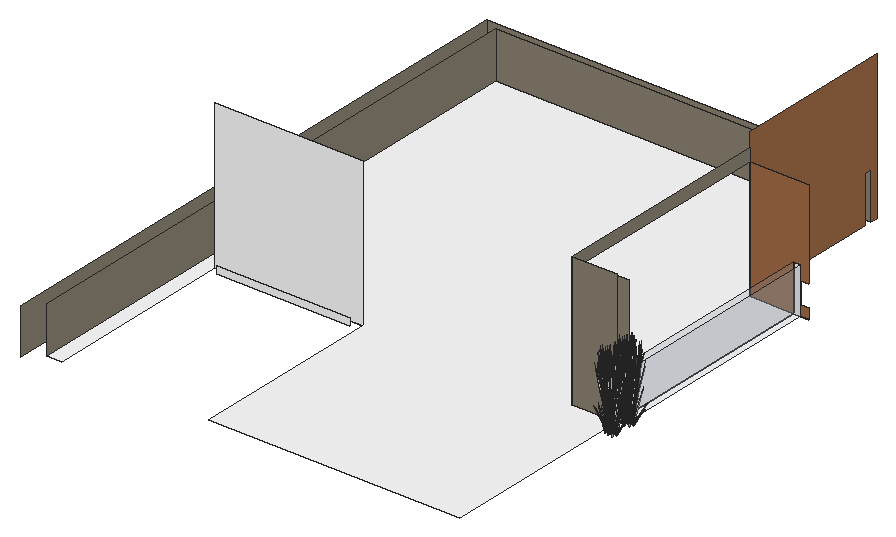
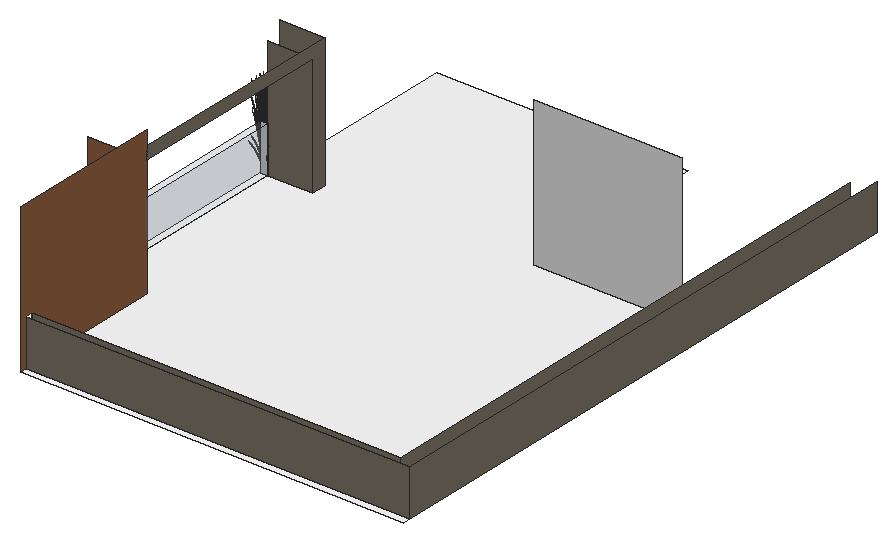
# SketchUp Ruby script. Lengths in inches.
U = 1.inch
M = Sketchup.active_model
def pt(a) = Geom::Point3d.new(a.map { |v| v * U })
def face(e, loops, mat)
  f = e.add_face(loops[0].map { |a| pt(a) })
  loops[1..].each { |l| e.add_face(l.map { |a| pt(a) }).erase! }
  f.material = f.back_material = mat if mat
  f
end
# faces: each face lists its corners as indices into pts; further lists are holes
def faces(e, pts, list, mat = nil) = list.each { |f| face(e, (f[0].is_a?(Array) ? f : [f]).map { |l| l.map { |i| pts[i] } }, mat) }
# xy, xz, yz: faces in a plane at the given z, y or x. An outline is a flat list of corners, or four numbers for a rectangle; further outlines are holes
def ring(l) = l.size == 4 ? [[l[0], l[1]], [l[2], l[1]], [l[2], l[3]], [l[0], l[3]]] : l.each_slice(2).to_a
def flat(e, list, mat, &to3) = list.each { |f| face(e, (f[0].is_a?(Array) ? f : [f]).map { |l| ring(l).map { |u, v| to3.(u, v) } }, mat) }
def xy(e, z, list, mat = nil) = flat(e, list, mat) { |x, y| [x, y, z] }
def xz(e, y, list, mat = nil) = flat(e, list, mat) { |x, z| [x, y, z] }
def yz(e, x, list, mat = nil) = flat(e, list, mat) { |y, z| [x, y, z] }
def lines(e, pts, list) = list.each { |a, b| e.add_line(pt(pts[a]), pt(pts[b])) }
# prism: a flat outline (further loops are holes) pulled along v
def prism(e, loops, v, mat = nil)
  f = face(e, loops, mat); d = Geom::Vector3d.new(v.map { |x| x * U })
  f.pushpull(f.normal.samedirection?(d) ? d.length : -d.length)
end
def box(e, o, s, mat = nil) = prism(e, [[o, [o[0] + s[0], o[1], o[2]], [o[0] + s[0], o[1] + s[1], o[2]], [o[0], o[1] + s[1], o[2]]]], [0, 0, s[2]], mat)
def at(x, y, z, deg = 0) = Geom::Transformation.translation(pt([x, y, z])) * Geom::Transformation.rotation(ORIGIN, Z_AXIS, deg.degrees)
def axes(o, x, y, z) = Geom::Transformation.new([*x, 0, *y, 0, *z, 0, *pt(o).to_a, 1])
def part(name) = M.definitions.add(name)
# library, detail: a bought-in or finely detailed component or shape, given as its bounding box
def library(name, o, s) = part(name).tap { |d| box(d.entities, o, s) }
def detail(e, o, s) = box(e.add_group.entities, o, s)
def put(e, d, t, mat = nil) = e.add_instance(d, t).tap { |i| i.material = mat if mat }
def group(e, t, mat = nil) = e.add_group.tap { |g| g.transformation = t; g.material = mat if mat }.entities
root = M.entities
M.materials.add("Glass_Basic_01").color = [183, 196, 211]
M.materials["Glass_Basic_01"].alpha = 0.23
M.materials.add("LightPink_Translucent").color = [144, 107, 117]
M.materials["LightPink_Translucent"].alpha = 0.75
M.materials.add("M00_Soft_Cloud").color = [255, 255, 255]
M.materials.add("Plaster_04_1K").color = [142, 132, 117]
M.materials.add("Wood_Veneer_15_1K").color = [163, 109, 71]
M.materials.add("[Color_007]1").color = [58, 58, 58]
c1 = part("blade")
p = [[2.15,0.21,22],[0,0.17,0],[0.09,0.45,0],[2.18,0.31,22],[2.29,0.31,22],[0.38,0.45,0],
  [2.48,0.24,33],[2.49,0.24,33],[2.48,0.22,33]]
faces(c1.entities,p,[[0,1,2,3],[4,5,2,3],[6,3,4,7],[8,0,3,6]])
c2 = part("seeds")
p = [[0.3,-0.1,1.38],[-0.01,-0.03,1.59],[-0.01,-0.03,0.03],[0.14,-0.07,-0.07],[0.29,-0.03,3],[0.15,0.01,3.11]]
faces(c2.entities,p,[[0,1,2,3],[1,0,4,5]],"LightPink_Translucent")
c3 = part("blade with seeds")
put(c3.entities,c1,at(0,0,0))
put(c3.entities,c2,axes([2.4,0.25,30.99],[1.5799,-0.05474,1.17369],[-0.12525,1.92788,0.29478],[-0.07173,-0.02425,1.56792]))
xy(root,255,[[60,75.98,72,75.98,72,231.98,192,231.98,192,75.98,396,75.98,396,234.98,360,234.98,360,246.98,396,246.98,396,414.98,360,414.98,360,531.98,60,531.98],[48,537.98,360,543.98]],"M00_Soft_Cloud")
xz(root,225.98,[[78,255,186,261]],"M00_Soft_Cloud")
xz(root,231.98,[[72,255,192,375]],"M00_Soft_Cloud")
xz(root,234.98,[[360,255,396,363]],"Plaster_04_1K")
xz(root,246.98,[[396,255,402,292.64]],"M00_Soft_Cloud")
xz(root,246.98,[[360,255,396,353]],"Plaster_04_1K")
xz(root,414.98,[[396,254.86,402,292.64],[402,254.86,408,255]],"M00_Soft_Cloud")
xz(root,414.98,[[360,255,396,255,396,292.64,402,292.64,402,280.64,408,280.64,408,352.79,360,352.79],[402,255,408,263.45]],"Wood_Veneer_15_1K")
xz(root,531.98,[[60,255,360,292.64]],"Plaster_04_1K")
xz(root,537.98,[[48,255,360,292.64]],"Plaster_04_1K")
yz(root,48,[[63.98,255,537.98,292.64]],"Plaster_04_1K")
yz(root,60,[[75.98,255,531.98,292.64]],"Plaster_04_1K")
yz(root,360,[[234.98,255,234.98,363,414.98,363,414.98,353,246.98,353,246.98,255]],"Plaster_04_1K")
yz(root,360,[[414.98,255,414.98,375,543.98,375,543.98,255,537.98,255,537.98,292.64,531.98,292.64,531.98,255]],"Wood_Veneer_15_1K")
yz(root,396,[[246.98,255,414.98,292.64]],"Glass_Basic_01")
yz(root,396,[[234.98,255,246.98,292.64]],"[Color_007]1")
yz(root,402,[[246.98,255,414.98,292.64]],"Glass_Basic_01")
p = [[396,414.98,254.86],[360,414.98,254.86]]
lines(root,p,[[0,1]])
put(root,c3,axes([403.3,218.62,257.1],[-0.31203,-0.62659,-0.69835],[0.89884,-0.22566,-0.18329],[-0.03449,-0.21218,1.54149]))
put(root,c3,axes([407.47,216.7,256.49],[-0.11372,-0.04814,1.76342],[-0.29211,-0.53779,-0.26939],[0.19706,-0.14594,0.30037]))
put(root,c3,axes([403.17,216.82,257.375],[-0.47504,-0.61229,0],[0.79476,-0.34146,-0.51607],[0.18101,-0.07777,1.63711]))
put(root,c3,axes([404.22,216.08,257.13],[-0.52505,0.35054,-0.03893],[-0.48109,-0.38392,-0.17649],[-0.03387,-0.10878,0.58215]))
put(root,c3,axes([401.46,218.53,257.02],[0,-0.61104,-0.49651],[0.85008,0,0],[0,-0.13917,1.57504]))
put(root,c3,axes([403.82,216.72,257.02],[0.7111,-0.30552,-0.49651],[0.42504,0.54784,0],[0.16196,-0.06958,1.57504]))
put(root,c3,axes([404.66,217.97,257.06],[0.51177,-0.45928,-0.62353],[0.63575,0.41646,-0.16365],[0.20507,-0.11457,1.37633]))
put(root,c3,axes([403.77,218.78,257.21],[0.36864,-0.55059,-0.44739],[0.76598,0.26498,0.21531],[0,-0.12692,1.43643]))
put(root,c3,axes([404.11,218.51,257.67],[-0.08854,-0.69723,-0.29095],[0.92215,-0.04216,-0.50002],[0.16238,-0.09287,1.59708]))
put(root,c3,axes([401.82,218.54,257.03],[0.53038,-0.38124,-0.30978],[0.53038,0.38124,0.30978],[0,-0.1228,1.38974]))
put(root,c3,axes([401.61,216.72,257.13],[-0.21918,0.49894,-0.03893],[-0.6746,-0.15348,-0.17649],[-0.10242,-0.08161,0.58215]))
put(root,c3,axes([403.68,219.24,257.67],[-0.85568,-0.29155,-0.29095],[0.41201,-0.61537,-0.50002],[-0.02689,-0.15109,1.59708]))
put(root,c3,axes([401.25,218.99,257.375],[-0.95008,0,0],[0,-0.68292,-0.51607],[0,-0.15554,1.63711]))
put(root,c3,axes([403.99,216.96,257.03],[0.70886,0.15119,-0.30978],[-0.17848,0.53243,0.30978],[0.1429,-0.0614,1.38974]))
put(root,c3,axes([401.98,218.8125,257.33],[-0.70674,0.51372,0.30756],[-0.70717,-0.50832,-0.36492],[-0.02468,-0.14589,1.64885]))
put(root,c3,axes([403.9,219.88,257.4375],[0.20138,-0.72405,-0.23429],[0.95485,0.12621,0.51271],[-0.16685,-0.09999,1.5644]))
put(root,c3,axes([406.67,216.97,257.375],[0.47504,-0.61229,0],[0.79476,0.34146,-0.51607],[0.18101,0.07777,1.63711]))
put(root,c3,axes([403.83,219.59,257.21],[-0.45644,-0.51287,-0.44739],[0.69137,-0.36116,0.21531],[-0.14771,-0.06346,1.43643]))
put(root,c3,axes([403.92,218.87,257.36],[0.33034,0.68327,0.45755],[-0.94388,0.2376,0.17955],[0.01154,-0.12555,1.58856]))
put(root,c3,axes([408.54,219.39,256.98],[-0.48937,0.07333,1.41583],[-0.07789,-0.58369,0.08104],[0.34275,-0.08835,0.80566]))
put(root,c3,axes([409.43,218.87,257.26],[-0.47106,-0.39072,-0.06488],[0.51591,-0.35801,-0.29416],[0.14618,-0.02521,0.97024]))
put(root,c3,axes([405.11,218.92,257.21],[0,-0.70701,0],[0.95008,0,0],[0,0,1.79456]))
put(root,c3,axes([403.42,219.79,257.06],[-0.79037,-0.10018,-0.62353],[0.16679,-0.61794,-0.16365],[-0.23587,-0.07488,1.37633]))
put(root,c3,axes([404.66,218.48,257.36],[-0.62999,0.55453,0.45755],[-0.74845,-0.4895,0.17955],[0.15188,-0.05534,1.58856]))
put(root,c3,axes([405.35,219.47,257.3],[-0.70674,-0.52593,-0.06131],[0.70717,-0.52625,0],[-0.02468,-0.01837,1.75571]))
put(root,c3,axes([403.24,218.06,256.59],[-0.74787,0.24464,1.28929],[-0.23804,-0.70192,0.50096],[0.45924,0.01168,1.46642]))
put(root,c3,axes([404.01,219.54,257.36],[0.96033,0.12874,0.45755],[-0.19544,0.7271,0.17955],[-0.14034,-0.07021,1.58856]))
put(root,c3,axes([409.08,219.01,256.49],[-0.03971,-0.09277,1.76342],[0.27541,-0.54264,-0.26939],[0.27782,-0.00781,0.30037]))
put(root,c3,axes([400.88,218.91,256.49],[0.01927,0.0963,1.76342],[-0.38846,0.5029,-0.26939],[-0.27592,-0.02535,0.30037]))
put(root,c3,axes([402.58,220.73,257.03],[-0.17848,-0.53243,-0.30978],[0.70886,-0.15119,0.30978],[-0.1429,-0.0614,1.38974]))
put(root,c3,axes([405.17,218.42,257.67],[0.76714,-0.40567,-0.29095],[0.51013,0.57321,-0.50002],[0.18927,0.05821,1.59708]))
put(root,c3,axes([402.38,220.96,257.02],[-0.7111,-0.30552,-0.49651],[0.42504,-0.54784,0],[-0.16196,-0.06958,1.57504]))
put(root,c3,axes([407.11,217.34,257.02],[0.7111,0.30552,-0.49651],[-0.42504,0.54784,0],[0.16196,0.06958,1.57504]))
put(root,c3,axes([405.76,219.08,257.21],[0.85008,0,0],[0,0.63259,0],[0,0,1.78407]))
put(root,c3,axes([404.32,219.88,257.67],[-0.76714,0.40567,-0.29095],[-0.51013,-0.57321,-0.50002],[-0.18927,-0.05821,1.59708]))
put(root,c3,axes([406.91,217.57,257.03],[0.17848,0.53243,-0.30978],[-0.70886,0.15119,0.30978],[0.1429,0.0614,1.38974]))
put(root,c3,axes([404.72,220.55,257.2],[-0.24791,-0.5268,0],[0.70791,-0.18448,0],[0,0,1.54371]))
put(root,c3,axes([405.64,220.48,257.18],[0.79769,-0.20732,-0.19198],[0.2803,0.59721,0.00008],[0.08805,-0.02292,1.73897]))
put(root,c3,axes([405.74,219.35,257.21],[0.53038,0.39469,0],[-0.53038,0.39469,0],[0,0,1.69266]))
put(root,c3,axes([406.07,218.51,257.06],[0.79037,0.10018,-0.62353],[-0.16679,0.61794,-0.16365],[0.23587,0.07488,1.37633]))
put(root,c3,axes([404.54,220.79,257.2],[-0.76598,-0.27433,0],[0.36864,-0.57001,0],[0,0,1.62707]))
put(root,c3,axes([405.18,220.0625,257.46],[-0.74193,-0.49181,-0.25192],[0.6243,-0.55226,0.5513],[-0.19979,0.05753,1.68216]))
put(root,c3,axes([405.59,219.21,257.29],[0,0.70667,-0.05637],[-0.95008,0,0],[0,0.02221,1.79368]))
put(root,c3,axes([405.66,218.7,257.21],[0.45644,0.51287,-0.44739],[-0.69137,0.36116,0.21531],[0.14771,0.06346,1.43643]))
put(root,c3,axes([402.82,221.32,257.375],[-0.47504,0.61229,0],[-0.79476,-0.34146,-0.51607],[-0.18101,-0.07777,1.63711]))
put(root,c3,axes([404.8,219.96,257.21],[-0.82508,0.03772,-0.44739],[-0.07462,-0.62614,0.21531],[-0.14771,0.06346,1.43643]))
put(root,c3,axes([405.41,220.8,257.2],[0.76598,0.27433,0],[-0.36864,0.57001,0],[0,0,1.74954]))
put(root,c3,axes([405.72,221.41,257.19],[-0.46912,-0.61443,-0.05142],[0.79476,-0.34146,0.51607],[-0.19584,0.0585,1.6363]))
put(root,c3,axes([405.13,220.57,257.29],[0.33034,0.70197,-0.06012],[-0.94388,0.24598,0],[0.01154,0.02451,1.72173]))
put(root,c3,axes([405.5,221.33,257.03],[-0.70886,-0.15119,-0.30978],[0.17848,-0.53243,0.30978],[-0.1429,0.0614,1.38974]))
put(root,c3,axes([408.24,219.3,257.375],[0.95008,0,0],[0,0.68292,-0.51607],[0,0.15554,1.63711]))
put(root,c3,axes([407.86,219.65,257.2],[-0.94962,-0.00489,-0.04976],[0,-0.68292,0.49943],[-0.02984,0.15546,1.58352]))
put(root,c3,axes([405.81,219.06,257.67],[0.85568,0.29155,-0.29095],[-0.41201,0.61537,-0.50002],[0.02689,0.15109,1.59708]))
put(root,c3,axes([407.67,219.75,257.03],[-0.53038,0.38124,-0.30978],[-0.53038,-0.38124,0.30978],[0,0.1228,1.38974]))
put(root,c3,axes([405.38,219.79,257.67],[0.08854,0.69723,-0.29095],[-0.92215,0.04216,-0.50002],[-0.16238,0.09287,1.59708]))
put(root,c3,axes([405.72,219.52,257.21],[-0.36864,0.55059,-0.44739],[-0.76598,-0.26498,0.21531],[0,0.12692,1.43643]))
put(root,c3,axes([404.83,220.32,257.06],[-0.51177,0.45928,-0.62353],[-0.63575,-0.41646,-0.16365],[-0.20507,0.11457,1.37633]))
put(root,c3,axes([405.74,221.09,257.33],[0.95122,0.19861,0.30756],[-0.23797,0.7099,-0.36492],[-0.15744,0.08885,1.64885]))
put(root,c3,axes([405.67,221.57,257.02],[-0.7111,0.30552,-0.49651],[-0.42504,-0.54784,0],[-0.16196,0.06958,1.57504]))
put(root,c3,axes([408.03,219.77,257.02],[0,0.61104,-0.49651],[-0.85008,0,0],[0,0.13917,1.57504]))
put(root,c3,axes([406.3125,221.48,257.375],[0.47504,0.61229,0],[-0.79476,0.34146,-0.51607],[-0.18101,0.07777,1.63711]))
put(root,c3,axes([407.07,221.69,256.49],[0.05536,-0.08822,1.76342],[0.69692,-0.25981,-0.26939],[0.21129,0.13447,0.30037]))
put(root,c3,axes([406.15,219.68,257.09],[0.2786,0.55945,-0.69212],[-0.80253,0.20149,-0.18165],[0.03079,0.18945,1.52773]))
put(root,c3,axes([400.67,221.61,256.49],[0.10192,0.06105,1.76342],[0.17281,0.56562,-0.26939],[-0.22588,0.12062,0.30037]))
put(root,c3,axes([403.82,221.67,256.49],[0.12297,-0.03325,1.76342],[0.73967,0.18301,-0.26939],[0.02163,0.20626,0.30037]))
put(root,c3,axes([404.51,232.72,256.49],[-0.12744,0.02202,1.76342],[-0.70477,-0.24781,-0.26939],[0.01183,-0.2067,0.30037]))
put(root,c3,axes([402.23,233.48,256.49],[-0.0736,0.08049,1.76342],[-0.74378,0.17355,-0.26939],[-0.17968,-0.15788,0.30037]))
put(root,c3,axes([403.46,235.6875,257.1],[-0.31203,-0.62659,-0.69835],[0.89884,-0.22566,-0.18329],[-0.03449,-0.21218,1.54149]))
put(root,c3,axes([407.63,233.77,256.49],[-0.11372,-0.04814,1.76342],[-0.29211,-0.53779,-0.26939],[0.19706,-0.14594,0.30037]))
put(root,c3,axes([403.33,233.89,257.375],[-0.47504,-0.61229,0],[0.79476,-0.34146,-0.51607],[0.18101,-0.07777,1.63711]))
put(root,c3,axes([404.375,233.15,257.13],[-0.52505,0.35054,-0.03893],[-0.48109,-0.38392,-0.17649],[-0.03387,-0.10878,0.58215]))
put(root,c3,axes([401.62,235.6,257.02],[0,-0.61104,-0.49651],[0.85008,0,0],[0,-0.13917,1.57504]))
put(root,c3,axes([403.98,233.79,257.02],[0.7111,-0.30552,-0.49651],[0.42504,0.54784,0],[0.16196,-0.06958,1.57504]))
put(root,c3,axes([404.82,235.04,257.06],[0.51177,-0.45928,-0.62353],[0.63575,0.41646,-0.16365],[0.20507,-0.11457,1.37633]))
put(root,c3,axes([403.93,235.85,257.21],[0.36864,-0.55059,-0.44739],[0.76598,0.26498,0.21531],[0,-0.12692,1.43643]))
put(root,c3,axes([404.27,235.58,257.67],[-0.08854,-0.69723,-0.29095],[0.92215,-0.04216,-0.50002],[0.16238,-0.09287,1.59708]))
put(root,c3,axes([401.98,235.61,257.03],[0.53038,-0.38124,-0.30978],[0.53038,0.38124,0.30978],[0,-0.1228,1.38974]))
put(root,c3,axes([401.77,233.79,257.13],[-0.21918,0.49894,-0.03893],[-0.6746,-0.15348,-0.17649],[-0.10242,-0.08161,0.58215]))
put(root,c3,axes([403.84,236.31,257.67],[-0.85568,-0.29155,-0.29095],[0.41201,-0.61537,-0.50002],[-0.02689,-0.15109,1.59708]))
put(root,c3,axes([401.4,236.0625,257.375],[-0.95008,0,0],[0,-0.68292,-0.51607],[0,-0.15554,1.63711]))
put(root,c3,axes([404.15,234.03,257.03],[0.70886,0.15119,-0.30978],[-0.17848,0.53243,0.30978],[0.1429,-0.0614,1.38974]))
put(root,c3,axes([402.14,235.88,257.33],[-0.70674,0.51372,0.30756],[-0.70717,-0.50832,-0.36492],[-0.02468,-0.14589,1.64885]))
put(root,c3,axes([404.05,236.95,257.4375],[0.20138,-0.72405,-0.23429],[0.95485,0.12621,0.51271],[-0.16685,-0.09999,1.5644]))
put(root,c3,axes([406.83,234.04,257.375],[0.47504,-0.61229,0],[0.79476,0.34146,-0.51607],[0.18101,0.07777,1.63711]))
put(root,c3,axes([403.99,236.66,257.21],[-0.45644,-0.51287,-0.44739],[0.69137,-0.36116,0.21531],[-0.14771,-0.06346,1.43643]))
put(root,c3,axes([404.08,235.9375,257.36],[0.33034,0.68327,0.45755],[-0.94388,0.2376,0.17955],[0.01154,-0.12555,1.58856]))
put(root,c3,axes([408.7,236.46,256.98],[-0.48937,0.07333,1.41583],[-0.07789,-0.58369,0.08104],[0.34275,-0.08835,0.80566]))
put(root,c3,axes([409.59,235.94,257.26],[-0.47106,-0.39072,-0.06488],[0.51591,-0.35801,-0.29416],[0.14618,-0.02521,0.97024]))
put(root,c3,axes([405.27,235.99,257.21],[0,-0.70701,0],[0.95008,0,0],[0,0,1.79456]))
put(root,c3,axes([403.58,236.86,257.06],[-0.79037,-0.10018,-0.62353],[0.16679,-0.61794,-0.16365],[-0.23587,-0.07488,1.37633]))
put(root,c3,axes([404.82,235.55,257.36],[-0.62999,0.55453,0.45755],[-0.74845,-0.4895,0.17955],[0.15188,-0.05534,1.58856]))
put(root,c3,axes([405.51,236.54,257.3],[-0.70674,-0.52593,-0.06131],[0.70717,-0.52625,0],[-0.02468,-0.01837,1.75571]))
put(root,c3,axes([403.39,235.125,256.59],[-0.74787,0.24464,1.28929],[-0.23804,-0.70192,0.50096],[0.45924,0.01168,1.46642]))
put(root,c3,axes([404.16,236.61,257.36],[0.96033,0.12874,0.45755],[-0.19544,0.7271,0.17955],[-0.14034,-0.07021,1.58856]))
put(root,c3,axes([409.24,236.08,256.49],[-0.03971,-0.09277,1.76342],[0.27541,-0.54264,-0.26939],[0.27782,-0.00781,0.30037]))
put(root,c3,axes([401.04,235.98,256.49],[0.01927,0.0963,1.76342],[-0.38846,0.5029,-0.26939],[-0.27592,-0.02535,0.30037]))
put(root,c3,axes([402.74,237.8,257.03],[-0.17848,-0.53243,-0.30978],[0.70886,-0.15119,0.30978],[-0.1429,-0.0614,1.38974]))
put(root,c3,axes([405.33,235.49,257.67],[0.76714,-0.40567,-0.29095],[0.51013,0.57321,-0.50002],[0.18927,0.05821,1.59708]))
put(root,c3,axes([402.54,238.03,257.02],[-0.7111,-0.30552,-0.49651],[0.42504,-0.54784,0],[-0.16196,-0.06958,1.57504]))
put(root,c3,axes([407.26,234.41,257.02],[0.7111,0.30552,-0.49651],[-0.42504,0.54784,0],[0.16196,0.06958,1.57504]))
put(root,c3,axes([405.91,236.15,257.21],[0.85008,0,0],[0,0.63259,0],[0,0,1.78407]))
put(root,c3,axes([404.47,236.95,257.67],[-0.76714,0.40567,-0.29095],[-0.51013,-0.57321,-0.50002],[-0.18927,-0.05821,1.59708]))
put(root,c3,axes([407.07,234.64,257.03],[0.17848,0.53243,-0.30978],[-0.70886,0.15119,0.30978],[0.1429,0.0614,1.38974]))
put(root,c3,axes([404.875,237.625,257.2],[-0.24791,-0.5268,0],[0.70791,-0.18448,0],[0,0,1.54371]))
put(root,c3,axes([405.8,237.55,257.18],[0.79769,-0.20732,-0.19198],[0.2803,0.59721,0.00008],[0.08805,-0.02292,1.73897]))
put(root,c3,axes([405.9,236.42,257.21],[0.53038,0.39469,0],[-0.53038,0.39469,0],[0,0,1.69266]))
put(root,c3,axes([406.23,235.58,257.06],[0.79037,0.10018,-0.62353],[-0.16679,0.61794,-0.16365],[0.23587,0.07488,1.37633]))
put(root,c3,axes([404.7,237.86,257.2],[-0.76598,-0.27433,0],[0.36864,-0.57001,0],[0,0,1.62707]))
put(root,c3,axes([405.34,237.13,257.46],[-0.74193,-0.49181,-0.25192],[0.6243,-0.55226,0.5513],[-0.19979,0.05753,1.68216]))
put(root,c3,axes([405.75,236.28,257.29],[0,0.70667,-0.05637],[-0.95008,0,0],[0,0.02221,1.79368]))
put(root,c3,axes([405.82,235.78,257.21],[0.45644,0.51287,-0.44739],[-0.69137,0.36116,0.21531],[0.14771,0.06346,1.43643]))
put(root,c3,axes([402.97,238.4,257.375],[-0.47504,0.61229,0],[-0.79476,-0.34146,-0.51607],[-0.18101,-0.07777,1.63711]))
put(root,c3,axes([404.96,237.03,257.21],[-0.82508,0.03772,-0.44739],[-0.07462,-0.62614,0.21531],[-0.14771,0.06346,1.43643]))
put(root,c3,axes([405.57,237.875,257.2],[0.76598,0.27433,0],[-0.36864,0.57001,0],[0,0,1.74954]))
put(root,c3,axes([405.875,238.48,257.19],[-0.46912,-0.61443,-0.05142],[0.79476,-0.34146,0.51607],[-0.19584,0.0585,1.6363]))
put(root,c3,axes([405.29,237.64,257.29],[0.33034,0.70197,-0.06012],[-0.94388,0.24598,0],[0.01154,0.02451,1.72173]))
put(root,c3,axes([405.66,238.4,257.03],[-0.70886,-0.15119,-0.30978],[0.17848,-0.53243,0.30978],[-0.1429,0.0614,1.38974]))
put(root,c3,axes([408.4,236.37,257.375],[0.95008,0,0],[0,0.68292,-0.51607],[0,0.15554,1.63711]))
put(root,c3,axes([408.02,236.72,257.2],[-0.94962,-0.00489,-0.04976],[0,-0.68292,0.49943],[-0.02984,0.15546,1.58352]))
put(root,c3,axes([405.97,236.13,257.67],[0.85568,0.29155,-0.29095],[-0.41201,0.61537,-0.50002],[0.02689,0.15109,1.59708]))
put(root,c3,axes([407.82,236.82,257.03],[-0.53038,0.38124,-0.30978],[-0.53038,-0.38124,0.30978],[0,0.1228,1.38974]))
put(root,c3,axes([405.54,236.86,257.67],[0.08854,0.69723,-0.29095],[-0.92215,0.04216,-0.50002],[-0.16238,0.09287,1.59708]))
put(root,c3,axes([405.875,236.59,257.21],[-0.36864,0.55059,-0.44739],[-0.76598,-0.26498,0.21531],[0,0.12692,1.43643]))
put(root,c3,axes([404.98,237.39,257.06],[-0.51177,0.45928,-0.62353],[-0.63575,-0.41646,-0.16365],[-0.20507,0.11457,1.37633]))
put(root,c3,axes([405.89,238.17,257.33],[0.95122,0.19861,0.30756],[-0.23797,0.7099,-0.36492],[-0.15744,0.08885,1.64885]))
put(root,c3,axes([405.83,238.64,257.02],[-0.7111,0.30552,-0.49651],[-0.42504,-0.54784,0],[-0.16196,0.06958,1.57504]))
put(root,c3,axes([408.1875,236.84,257.02],[0,0.61104,-0.49651],[-0.85008,0,0],[0,0.13917,1.57504]))
put(root,c3,axes([406.47,238.55,257.375],[0.47504,0.61229,0],[-0.79476,0.34146,-0.51607],[-0.18101,0.07777,1.63711]))
put(root,c3,axes([407.23,238.76,256.49],[0.05536,-0.08822,1.76342],[0.69692,-0.25981,-0.26939],[0.21129,0.13447,0.30037]))
put(root,c3,axes([406.31,236.75,257.09],[0.2786,0.55945,-0.69212],[-0.80253,0.20149,-0.18165],[0.03079,0.18945,1.52773]))
put(root,c3,axes([400.83,238.68,256.49],[0.10192,0.06105,1.76342],[0.17281,0.56562,-0.26939],[-0.22588,0.12062,0.30037]))
put(root,c3,axes([403.97,238.74,256.49],[0.12297,-0.03325,1.76342],[0.73967,0.18301,-0.26939],[0.02163,0.20626,0.30037]))
